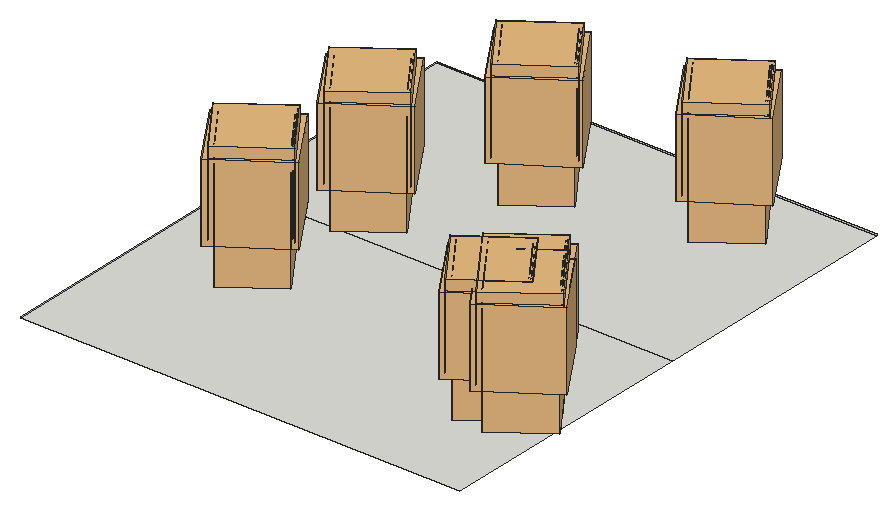
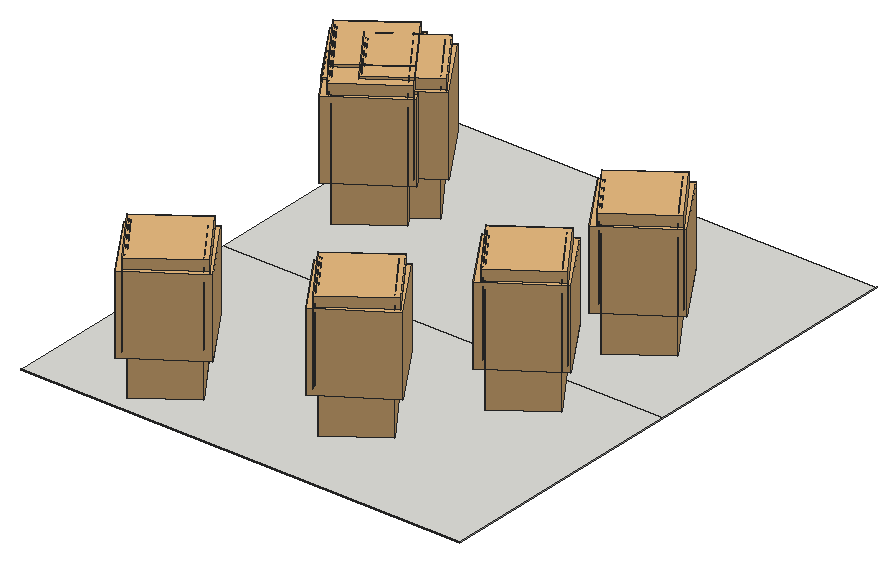
# SketchUp Ruby script. Lengths in inches.
U = 1.inch
M = Sketchup.active_model
def pt(a) = Geom::Point3d.new(a.map { |v| v * U })
def face(e, loops, mat)
  f = e.add_face(loops[0].map { |a| pt(a) })
  loops[1..].each { |l| e.add_face(l.map { |a| pt(a) }).erase! }
  f.material = f.back_material = mat if mat
  f
end
# faces: each face lists its corners as indices into pts; further lists are holes
def faces(e, pts, list, mat = nil) = list.each { |f| face(e, (f[0].is_a?(Array) ? f : [f]).map { |l| l.map { |i| pts[i] } }, mat) }
# xy, xz, yz: faces in a plane at the given z, y or x. An outline is a flat list of corners, or four numbers for a rectangle; further outlines are holes
def ring(l) = l.size == 4 ? [[l[0], l[1]], [l[2], l[1]], [l[2], l[3]], [l[0], l[3]]] : l.each_slice(2).to_a
def flat(e, list, mat, &to3) = list.each { |f| face(e, (f[0].is_a?(Array) ? f : [f]).map { |l| ring(l).map { |u, v| to3.(u, v) } }, mat) }
def xy(e, z, list, mat = nil) = flat(e, list, mat) { |x, y| [x, y, z] }
def xz(e, y, list, mat = nil) = flat(e, list, mat) { |x, z| [x, y, z] }
def yz(e, x, list, mat = nil) = flat(e, list, mat) { |y, z| [x, y, z] }
def lines(e, pts, list) = list.each { |a, b| e.add_line(pt(pts[a]), pt(pts[b])) }
# prism: a flat outline (further loops are holes) pulled along v
def prism(e, loops, v, mat = nil)
  f = face(e, loops, mat); d = Geom::Vector3d.new(v.map { |x| x * U })
  f.pushpull(f.normal.samedirection?(d) ? d.length : -d.length)
end
def box(e, o, s, mat = nil) = prism(e, [[o, [o[0] + s[0], o[1], o[2]], [o[0] + s[0], o[1] + s[1], o[2]], [o[0], o[1] + s[1], o[2]]]], [0, 0, s[2]], mat)
def at(x, y, z, deg = 0) = Geom::Transformation.translation(pt([x, y, z])) * Geom::Transformation.rotation(ORIGIN, Z_AXIS, deg.degrees)
def axes(o, x, y, z) = Geom::Transformation.new([*x, 0, *y, 0, *z, 0, *pt(o).to_a, 1])
def part(name) = M.definitions.add(name)
# library, detail: a bought-in or finely detailed component or shape, given as its bounding box
def library(name, o, s) = part(name).tap { |d| box(d.entities, o, s) }
def detail(e, o, s) = box(e.add_group.entities, o, s)
def put(e, d, t, mat = nil) = e.add_instance(d, t).tap { |i| i.material = mat if mat }
def group(e, t, mat = nil) = e.add_group.tap { |g| g.transformation = t; g.material = mat if mat }.entities
root = M.entities
M.materials.add("028_190k_fullGeometry_Material \#4").color = [120, 148, 64]
M.materials.add("Colorsadfasdfa0sd1f06w3").color = [153, 130, 61]
M.materials.add("Euphorbia asdfasd0f150160s159w").color = [180, 173, 131]
M.materials.add("Euphorbiaasdfa0sdf1a56sd016wow Leaf SU").color = [141, 134, 72]
M.materials.add("asdfasdf0165f6asdLeafVar1sfd015as60f1as6").color = [231, 235, 211]
M.materials.add("dw_stemssadfasdfa0sdf1s01d6w1").color = [90, 97, 50]
M.materials.add("viburnumblaasdfas0df1w06d").color = [98, 102, 84]
M.materials.add("viburnumbladsadfasdfad0w122").color = [125, 129, 119]
c1 = part("Component\#315")
p = [[0.25,0,0],[2.05,0.01,0.35],[1.81,4.2,1.66],[0,4.19,1.3125]]
faces(c1.entities,p,[[0,1,2,3]],"viburnumbladsadfasdfad0w122")
c2 = part("viburnumblad2")
put(c2.entities,c1,axes([-19.23,-4.49,-32.18],[83.35428,0,0],[0,79.38502,0],[0,0,83.35428]))
c3 = part("vdw_leaf\#3")
p = [[0,0,0],[-2.77,1.61,2.32],[-4.3125,6.1,4.5],[-3.97,13.49,6.09],[-2.47,18.57,6.3],[-0.2,22.73,5.75],
  [2.54,19.66,6.85],[4.3,15.93,7.09],[5.03,7.6,5.43],[3.32,1.76,2.74]]
faces(c3.entities,p,[[0,1,2,3,4,5],[0,5,6,7,8,9]],"asdfasdf0165f6asdLeafVar1sfd015as60f1as6")
c4 = part("dw_brancj_2\#2")
p = [[9.7,-0.22,29.95],[0.23,-1.96,0.34],[-0.05,1.51,0.11],[9.65,1.51,29.46],[18.64,-8.75,84.43],[18.96,-6.63,84.625],
  [1.53,6.02,63.68],[1.42,8.18,63.25],[-10.58,8.77,161.17],[-10.41,9.98,160.68],[26.34,-9.37,211.72],[26.57,-8.28,211.23]]
faces(c4.entities,p,[[0,1,2],[0,2,3],[4,0,3],[4,3,5],[6,0,3],[6,3,7],[8,6,7],[8,7,9],
  [10,4,5],[10,5,11]],"dw_stemssadfasdfa0sdf1s01d6w1")
c5 = part("vdw_branch2\#3")
put(c5.entities,c3,axes([19.53,-5.9,102.42],[1.12377,-0.50004,0],[0.46097,1.03596,0.47664],[-0.19377,-0.43548,1.13389]))
put(c5.entities,c3,axes([-5.89,6.52,109.44],[-1.07209,0.83679,0],[-0.77141,-0.98832,0.52702],[0.32427,0.41545,1.25373]))
put(c5.entities,c3,axes([-0.44,8.23,75.28],[0.88709,-0.9947,0],[0.92159,0.82189,0.33087],[-0.25219,-0.22491,1.26111]))
put(c5.entities,c3,axes([24.71,-8.97,190.81],[-0.82641,0.91101,0],[-0.83983,-0.76184,0.47664],[0.35303,0.32025,1.13389]))
put(c5.entities,c3,axes([-2.29,8.24,91.35],[1.24603,-0.47303,0],[0.43826,1.15445,0.33087],[-0.11993,-0.31592,1.26111]))
put(c5.entities,c3,axes([12.26,-3.11,37.92],[-0.64625,1.02205,0.22511],[-1.04383,-0.61044,-0.22511],[-0.07533,-0.30931,1.18809]))
put(c5.entities,c3,axes([26.17,-9.17,210.27],[-0.99452,-0.10453,0],[0.09636,-0.91681,0.38752],[-0.04051,0.38539,0.92186]))
put(c5.entities,c3,axes([-6.07,9.4,125.35],[-0.90214,-0.98107,0],[0.90896,-0.83583,0.33087],[-0.24874,0.22873,1.26111]))
put(c5.entities,c3,axes([-4.13,7.29,110.58],[0.44715,-1.078,0.64369],[1.05816,0.63649,0.33087],[-0.58725,0.40856,1.09216]))
put(c5.entities,c3,axes([23.91,-8.22,171.96],[0.62307,0.85009,-0.63406],[-0.71531,0.8798,0.47664],[0.78296,0.12729,0.94004]))
put(c5.entities,c4,at(-0.09,0.18,-0.25),"dw_stemssadfasdfa0sdf1s01d6w1")
put(c5.entities,c3,axes([23.34,-9.65,156.59],[-0.31364,-1.00782,0.58216],[1.10369,-0.17062,0.29925],[-0.17137,0.6239,0.98776]))
put(c5.entities,c3,axes([15.03,-3.37,58.83],[-1.05425,-0.00194,0.58442],[-0.14303,-1.11707,-0.26172],[0.55355,-0.3046,0.99755]))
put(c5.entities,c3,axes([-11.625,9.46,160.37],[0.36812,0.92978,0],[-0.85713,0.33936,0.38752],[0.3603,-0.14265,0.92186]))
put(c5.entities,c3,axes([21.32,-8.53,138.72],[1.21379,0.19904,0],[-0.19904,1.21379,0],[0,0,1.23]))
put(c5.entities,c3,axes([22.54,-9.2,141.43],[-1.02887,0.17955,0.60182],[-0.23387,-1.13057,-0.06253],[0.56696,-0.17376,1.02111]))
put(c5.entities,c3,axes([23.9,-8.82,173.84],[-1.14567,-0.37474,0],[0.35918,-1.0981,0.04438],[-0.01409,0.04308,1.17993]))
put(c5.entities,c3,axes([-7.84,8.92,143.59],[-1.26971,0.40522,0],[-0.37543,-1.17638,0.33087],[0.10274,0.32192,1.26111]))
put(c5.entities,c3,axes([19.77,-8.01,85.98],[-0.32405,-1.14591,0.18674],[1.10278,-0.32969,-0.10948],[0.15845,0.14442,1.16117]))
put(c5.entities,c3,axes([-0.62,5.76,76.34],[-0.08879,1.17576,-0.67771],[-1.34525,-0.16582,-0.11144],[-0.17897,0.66309,1.17383]))
put(c5.entities,c3,axes([20.49,-8.22,121.07],[0.39924,-0.78471,-0.8233],[1.08735,0.33121,0.2116],[0.09035,-0.83005,0.83495]))
put(c5.entities,c3,axes([15.15,-3.72,62.9],[1.16251,0.40128,-0.0211],[-0.39924,1.16074,0.07874],[0.0456,-0.06757,1.2273]))
put(c5.entities,c3,axes([20.72,-8.08,120.26],[-0.03693,1.2277,-0.06551],[-1.22944,-0.03698,0],[-0.00197,0.06548,1.22825]))
put(c5.entities,c3,axes([22.58,-8.36,155.57],[-0.56247,1.09386,0],[-1.00839,-0.51852,0.47664],[0.42389,0.21796,1.13389]))
put(c5.entities,c3,axes([3.97,3.13,57.96],[-1.09459,0.76041,0],[-0.72262,-1.0402,-0.1735],[-0.10109,-0.14552,1.29352]))
put(c5.entities,c3,axes([-10.8,9.06,160.75],[-0.66334,-0.72138,0],[0.66835,-0.61458,0.24329],[-0.1829,0.16818,0.92729]))
put(c5.entities,c3,axes([19.06,-9.3125,103.96],[-1.01345,0.25553,-0.60051],[-0.2265,-1.12952,-0.09839],[-0.59598,0.03076,1.01889]))
put(c5.entities,c3,axes([18.07,-6.2,81.7],[-0.56247,1.09386,0],[-1.00839,-0.51852,0.47664],[0.42389,0.21796,1.13389]))
put(c5.entities,c3,axes([12.95,-0.39,43.31],[0.13044,-1.19832,0],[1.11025,0.12085,0.29925],[-0.30382,-0.03307,1.14057]))
put(c5.entities,c3,axes([2.28,8.28,56.18],[1.32413,-0.31027,0],[0.30923,1.31968,-0.11144],[0.02542,0.1085,1.35543]))
put(c5.entities,c3,axes([-7.55,9.96,143.07],[1.34251,-0.21744,0],[0.20045,1.23761,0.52702],[-0.08426,-0.52024,1.25373]))
put(c5.entities,c3,axes([26.15,-8.25,210.66],[0.94661,-0.25364,0],[0.235,0.87703,0.24329],[-0.06431,-0.24,0.92729]))
put(c5.entities,c3,axes([-6.48,11.37,125.16],[0.64635,1.10315,0.46356],[-1.16569,0.46153,0.52702],[0.27017,-0.6478,1.16488]))
put(c5.entities,c3,axes([25.74,-8.35,191.28],[0.13044,-1.19832,0],[1.11025,0.12085,0.29925],[-0.30382,-0.03307,1.14057]))
put(c5.entities,c3,axes([-5.125,7.47,91.6],[-1.10024,0.63688,0.48318],[-0.78682,-1.00808,-0.46292],[0.14137,-0.65404,1.184]))
c6 = part("Component\#314")
p = [[0.14,0,0],[2.58,0.05,0.25],[2.44,5.11,2.64],[0,5.05,2.39]]
faces(c6.entities,p,[[0,1,2,3]],"viburnumblaasdfas0df1w06d")
c7 = part("viburnumblad1\#2")
put(c7.entities,c6,axes([-37.25,6.23,19.31],[75.98784,0,0],[0,65.50676,0],[0,0,75.98784]))
c8 = part("vdw_leaf\#2")
p = [[0,0,0],[-2.77,1.61,2.32],[-4.3125,6.1,4.5],[-3.97,13.49,6.09],[-2.47,18.57,6.3],[-0.2,22.73,5.75],
  [2.54,19.66,6.85],[4.3,15.93,7.09],[5.03,7.6,5.43],[3.32,1.76,2.74]]
faces(c8.entities,p,[[0,1,2,3,4,5],[0,5,6,7,8,9]],"asdfasdf0165f6asdLeafVar1sfd015as60f1as6")
c9 = part("dg_branch_1\#2")
p = [[46.12,1.57,35.62],[46,5.42,35.41],[0.14,1.79,0.05],[0.26,-2.0625,0.27],[74.05,2.99,75.8],[74.11,5.28,75.58],
  [103.46,0.47,94.74],[104.03,2.92,94.84],[81.14,16.92,120.46],[81.2,18.78,120.24],[130.47,-5.6875,130.27],[130.58,-3.66,129.85],
  [80.82,34.4375,191.22],[80.64,35.93,190.9],[148.49,-14.56,203.24],[148.9,-12.8125,203.11],[81.08,37.95,226.93],[81.4,39.1,227.03],
  [157.45,-18.19,250.77],[157.7,-17.01,250.41]]
faces(c9.entities,p,[[0,1,2,3],[4,0,1],[4,1,5],[6,4,5],[6,5,7],[8,4,5],[8,5,9],[10,6,7],
  [10,7,11],[12,8,9],[12,9,13],[14,10,11],[14,11,15],[16,12,13],[16,13,17],[18,14,15],
  [18,15,19]],"dw_stemssadfasdfa0sdf1s01d6w1")
c10 = part("vdw_branch1\#3")
put(c10.entities,c8,axes([120.69,-2.42,117.31],[1.12221,-0.24063,-0.65809],[0.19207,1.24776,-0.12871],[0.65778,0.01392,1.11658]))
put(c10.entities,c8,axes([81,38.9,226.05],[0.7888,-0.58155,0],[0.48308,0.65523,0.47],[-0.28484,-0.38635,0.83138]))
put(c10.entities,c8,axes([78.08,12.69,106.05],[-1.43826,-0.02353,-0.03177],[0.0088,-1.31777,0.57755],[-0.03854,0.57714,1.31741]))
put(c10.entities,c8,axes([130.18,-4.73,130.41],[-0.38031,-1.29044,-0.11242],[1.20662,-0.31032,-0.51987],[0.47109,-0.24694,1.24081]))
put(c10.entities,c8,axes([157.08,-17.89,249.93],[-0.91355,0.40674,0],[-0.37496,-0.84216,0.38752],[0.15762,0.35401,0.92186]))
put(c10.entities,c8,axes([90.64,3.03,86.49],[0.32514,-0.85045,-0.99675],[0.69523,0.98247,-0.61148],[1.11061,-0.36604,0.67459]))
put(c10.entities,c8,axes([80.15,28.42,160.95],[-0.16039,0.95636,-1.06292],[-1.41646,0.03966,0.24943],[0.19509,1.07422,0.93709]))
put(c10.entities,c8,axes([126.74,-5.45,129.22],[-0.59819,0.96152,-0.6841],[-0.85772,0.12575,0.92675],[0.75427,0.88089,0.57856]))
put(c10.entities,c8,axes([133.22,-6.12,150.66],[-0.93823,0.76985,0.59124],[-0.47726,-1.08188,0.65135],[0.84525,0.24366,1.02405]))
put(c10.entities,c8,axes([80.43,22.89,141.32],[-1.42571,-0.19312,0.01373],[0.18338,-1.31425,0.5561],[-0.0621,0.5528,1.32692]))
put(c10.entities,c8,axes([33.14,0.88,26.42],[-0.13338,1.31536,0.04876],[-1.04528,-0.13221,0.7073],[0.72315,0.03348,1.07497]))
put(c10.entities,c8,axes([152.63,-15.08,221.76],[-1.28188,0.41945,0.0579],[-0.3638,-1.18547,0.53367],[0.21665,0.49113,1.23869]))
put(c10.entities,c8,axes([80.05,28.28,160.33],[-0.46732,-1.26661,0.40679],[1.27397,-0.40257,0.21004],[-0.07408,0.44645,1.30501]))
put(c10.entities,c8,axes([153.95,-14.8,235.875],[0.39005,1.07743,0.20605],[-0.96443,0.25296,0.50293],[0.42961,-0.3464,0.99807]))
put(c10.entities,c8,axes([80.2,24.22,141.74],[1.33062,-0.46576,0.02628],[0.44746,1.2746,-0.06608],[-0.00197,0.0722,1.37936]))
put(c10.entities,c8,axes([145.48,-12.5,188.92],[-1.32952,0.16983,0.16138],[-0.09299,-1.2361,0.53471],[0.21503,0.51548,1.22904]))
put(c10.entities,c8,axes([139.64,-9.18,171.24],[0.05682,1.30088,0.23414],[-1.13176,-0.05343,0.57151],[0.58357,-0.22963,1.13417]))
put(c10.entities,c8,axes([70.95,4.35,71.98],[-1.1081,-0.41873,0.64752],[0.33675,-1.28259,-0.25313],[0.6937,-0.04625,1.15721]))
put(c10.entities,c8,axes([59.85,4.55,56.17],[-0.26797,1.24526,0.35754],[-0.9369,-0.41634,0.74783],[0.83377,-0.10389,0.98674]))
put(c10.entities,c8,axes([33.11,3.36,25.66],[-0.57817,-1.07968,-0.5679],[1.11554,-0.21356,-0.7297],[0.49375,-0.78178,0.98363]))
put(c10.entities,c9,at(-0.21,0.34,-0.17),"dw_stemssadfasdfa0sdf1s01d6w1")
put(c10.entities,c8,axes([80.91,19.01,122.53],[-0.84258,1.13222,-0.27981],[-1.15093,-0.75138,0.42537],[0.18861,0.47293,1.3457]))
put(c10.entities,c8,axes([119.8,-1.22,114.1],[-1.3235,-0.25012,0.09101],[0.25933,-1.31572,0.15537],[0.05991,0.1698,1.33794]))
put(c10.entities,c8,axes([46.29,5.1,38.04],[0.98937,0.73827,-0.47585],[-0.72359,1.03721,0.10473],[0.44068,0.18581,1.20453]))
put(c10.entities,c8,axes([81.1875,33.03,184.45],[1.33883,0.26986,0.35053],[-0.09581,1.22087,-0.57399],[-0.42216,0.53228,1.20262]))
put(c10.entities,c8,axes([80.16,36.28,206.98],[-0.83993,0.85737,-0.6234],[-1.05964,-0.65701,0.5241],[0.02941,0.81391,1.07976]))
put(c10.entities,c8,axes([154.86,-16.15,234.87],[0.02509,-1.15302,-0.28506],[1.1487,-0.04894,0.29908],[-0.30202,-0.28195,1.11384]))
put(c10.entities,c8,axes([108.77,-0.33,101.14],[-0.47691,-1.03266,-0.72709],[1.25395,-0.29455,-0.40416],[0.15052,-0.81814,1.06325]))
put(c10.entities,c8,axes([89.79,3.01,85.87],[-0.61344,0.75518,0.8965],[-0.17758,-1.01824,0.73622],[1.13385,0.22574,0.58569]))
put(c10.entities,c8,axes([81.56,20.31,123.29],[0.37259,-1.3435,0.21057],[1.29385,0.32364,-0.22445],[0.16906,0.25791,1.34638]))
put(c10.entities,c8,axes([46.45,1.82,36.74],[-0.77883,0.29892,1.0614],[0.19124,-1.24314,0.49044],[1.08598,0.43329,0.67484]))
put(c10.entities,c8,axes([71.37,4.02,72.32],[0.72905,0.81546,-0.74421],[-0.66805,0.98958,0.42988],[0.8391,0.14186,0.97745]))
put(c10.entities,c8,axes([136.59,-5.88,150.53],[0.85845,-0.99897,-0.12437],[0.96526,0.81273,0.13453],[-0.02572,-0.18182,1.28292]))
put(c10.entities,c8,axes([80.375,38.8,225.86],[-0.25178,0.96778,0],[-0.89216,-0.23211,0.38752],[0.37503,0.09757,0.92186]))
put(c10.entities,c8,axes([74.43,7.99,85.38],[-1.05703,0.91669,-0.33543],[-0.95806,-0.87958,0.61531],[0.18697,0.6754,1.25659]))
put(c10.entities,c8,axes([76.57,9.74,89.32],[0.63146,-1.21538,0.33508],[1.18148,0.49387,-0.43517],[0.26321,0.48577,1.26593]))
put(c10.entities,c8,axes([81.6875,36.97,207.4],[0.09422,-1.04424,0.38486],[1.01646,0.1939,0.27727],[-0.33299,0.33382,0.98727]))
put(c10.entities,c8,axes([157.29,-17.17,249.98],[0.50586,-0.50586,0],[0.38853,0.38853,0.41105],[-0.29684,-0.29684,0.56115]))
put(c10.entities,c8,axes([79.92,15.8,106.09],[1.03917,-0.29343,-0.90675],[-0.14587,1.22131,-0.5624],[0.92163,0.5191,0.88824]))
put(c10.entities,c8,axes([61.95,3.88,56.26],[0.41243,-1.28546,0],[1.17466,0.37688,-0.54831],[0.5221,0.16751,1.23363]))
put(c10.entities,c8,axes([151.99,-14.79,208.15],[-0.48571,-1.21723,-0.32393],[1.25386,-0.50033,0],[-0.12005,-0.30087,1.31056]))
put(c10.entities,c8,axes([108.44,0.62,102.22],[0.82183,0.96078,0.38967],[-0.62327,0.08618,1.10203],[0.79141,-0.88661,0.51693]))
put(c10.entities,c8,axes([145.6,-10.56,188.62],[1.03241,-0.02554,-0.82693],[0.3944,1.11584,0.45794],[0.70325,-0.61672,0.89706]))
put(c10.entities,c8,axes([78.59,32.3,183.89],[-1.12675,-0.42036,0.43987],[0.5899,-0.98149,0.57312],[0.14901,0.70693,1.05726]))
put(c10.entities,c8,axes([152.08,-13.42,223.37],[0.79993,-0.44251,-0.69938],[0.68456,0.82615,0.26026],[0.41048,-0.60953,0.85515]))
put(c10.entities,c8,axes([140.71,-8.74,170.55],[0.41903,-1.24177,-0.32393],[1.26224,0.33728,0.33986],[-0.23168,-0.40836,1.26573]))
put(c10.entities,c8,axes([149.25,-12.53,205.78],[1.24456,0.38285,0.23414],[-0.42999,1.04826,0.57151],[-0.02056,-0.62679,1.13417]))
c11 = part("Component\#306")
p = [[4.55,0.11,0],[4.55,0,0],[2.84,0,3.13],[2.84,0.11,3.13],[4.625,0.05,0.04],[2.92,0.05,3.15],
  [2.08,0,8.07],[2.08,0.11,8.07],[2.16,0.05,8.1],[0,0,12.54],[0,0.11,12.54],[0.07,0.05,12.58]]
faces(c11.entities,p,[[0,1,2,3],[1,4,5,2],[1,0,4],[4,0,3,5],[3,2,6,7],[2,5,8,6],[5,3,7,8],[7,6,9,10],
  [6,8,11,9],[8,7,10,11],[10,9,11]],"Colorsadfasdfa0sd1f06w3")
c12 = part("Component\#301")
xy(c12.entities,0,[[0,0,0.7,3.1]],"Euphorbiaasdfa0sdf1a56sd016wow Leaf SU")
c13 = part("Leaf rosette")
put(c13.entities,c12,axes([2.21,1.74,0.13],[-0.4441,0.47879,-0.0956],[-0.4878,-0.4406,0.05935],[-0.03146,0.16757,0.98536]))
put(c13.entities,c12,axes([2.29,1.9,0.17],[-0.62678,-0.10063,-0.18061],[0.01105,-0.59203,0.2915],[-0.31282,0.41486,0.85442]))
put(c13.entities,c12,axes([2.09,1.69,0.1],[-0.10438,0.65169,0],[-0.65169,-0.10438,0],[0,0,1]))
put(c13.entities,c12,axes([1.97,1.77,0.02],[0.31114,0.5228,0.25587],[-0.57125,0.32993,0.02052],[-0.16918,-0.3502,0.92127]))
put(c13.entities,c12,axes([1.93,1.95,0],[0.54816,-0.03215,0.36617],[-0.11878,0.60671,0.23108],[-0.52706,-0.39065,0.75472]))
put(c13.entities,c12,axes([2.04,2.1,0.05],[0.26275,-0.55867,0.23335],[0.34186,0.34684,0.44545],[-0.75711,-0.08556,0.64766]))
put(c13.entities,c12,axes([2.22,2.08,0.13],[-0.29265,-0.59104,-0.02512],[0.40323,-0.2198,0.47401],[-0.65583,0.2952,0.69479]))
c14 = part("Component\#308")
xy(c14.entities,0,[[0,0,5.01,4.64]],"Euphorbia asdfasd0f150160s159w")
c15 = part("Component\#316")
put(c15.entities,c11,at(2.35,3.5,0))
put(c15.entities,c13,at(0.25,1.59,12.45))
put(c15.entities,c14,axes([7.46,0.77,3.64],[0.10848,0.99337,0.03799],[-0.82378,0.11122,-0.55589],[-0.55643,0.02901,0.83038]))
put(c15.entities,c14,axes([1.97,2.58,1.93],[0.80762,-0.50565,0.30344],[0.47433,0.86274,0.17519],[-0.35038,0.00244,0.93661]))
put(c15.entities,c14,axes([5.79,0.14,3.9],[0.5013,0.78918,0.35482],[-0.74775,0.60146,-0.2813],[-0.4354,-0.1243,0.89162]))
put(c15.entities,c14,axes([1.87,2.6,3.75],[0.73154,-0.49698,0.46676],[0.47433,0.86274,0.17519],[-0.48976,0.09324,0.86686]))
put(c15.entities,c14,axes([3.91,7.06,6.66],[-0.50827,-0.83837,-0.19699],[0.8278,-0.53869,0.15675],[-0.23753,-0.08339,0.96779]))
put(c15.entities,c14,axes([1.2,3.99,6.83],[0.56066,-0.79708,0.22433],[0.74237,0.60386,0.29025],[-0.36682,0.0038,0.93028]))
put(c15.entities,c12,axes([2.42,3.73,12.57],[-0.1322,-0.64472,0.04955],[0.10064,0.02944,0.65162],[-0.9678,0.2092,0.14002]))
put(c15.entities,c12,axes([2.57,3.43,12.63],[-0.62833,0.089,-0.18134],[-0.19954,-0.36568,0.51192],[-0.04764,0.82148,0.56824]))
put(c15.entities,c14,axes([4.04,6.92,11.09],[-0.67411,-0.5063,-0.5378],[0.44628,-0.85937,0.24964],[-0.58857,-0.07172,0.80526]))
put(c15.entities,c12,axes([2.5,3.49,12.74],[-0.62833,0.089,-0.18134],[-0.18746,-0.03618,0.63178],[0.11402,0.98935,0.09049]))
put(c15.entities,c12,axes([2.3,3.27,12.51],[0.02916,0.64747,0.12464],[-0.56235,-0.04072,0.34308],[0.5216,-0.18387,0.83314]))
put(c15.entities,c14,axes([0.26,4.96,9.69],[0.33661,-0.92735,0.16343],[0.73504,0.36725,0.56995],[-0.58857,-0.07172,0.80526]))
put(c15.entities,c14,axes([4.76,6.31,12.62],[-0.95056,-0.1129,-0.28929],[0.09021,-0.99179,0.09066],[-0.29715,0.06008,0.95294]))
put(c15.entities,c14,axes([5.2,6.55,10.37],[-0.76372,-0.27738,-0.58291],[0.26517,-0.95808,0.10848],[-0.58857,-0.07172,0.80526]))
c16 = part("Plant stem")
p = [[2.84,0.11,3.13],[2.84,0,3.13],[2.08,0,8.07],[2.08,0.11,8.07],[2.92,0.05,3.15],[2.16,0.05,8.1],
  [0,0,12.54],[0,0.11,12.54],[0.07,0.05,12.58]]
faces(c16.entities,p,[[0,1,2,3],[1,4,5,2],[4,0,3,5],[3,2,6,7],[2,5,8,6],[5,3,7,8],[7,6,8]],"Colorsadfasdfa0sd1f06w3")
c17 = part("Leafy shoot")
put(c17.entities,c16,at(2.35,3.5,0))
put(c17.entities,c13,at(0.25,1.59,12.45))
put(c17.entities,c14,axes([1.87,2.6,3.75],[0.73154,-0.49698,0.46676],[0.47433,0.86274,0.17519],[-0.48976,0.09324,0.86686]))
put(c17.entities,c14,axes([3.91,7.06,6.66],[-0.50827,-0.83837,-0.19699],[0.8278,-0.53869,0.15675],[-0.23753,-0.08339,0.96779]))
put(c17.entities,c14,axes([1.2,3.99,6.83],[0.56066,-0.79708,0.22433],[0.74237,0.60386,0.29025],[-0.36682,0.0038,0.93028]))
put(c17.entities,c12,axes([2.42,3.73,12.57],[-0.1322,-0.64472,0.04955],[0.10064,0.02944,0.65162],[-0.9678,0.2092,0.14002]))
put(c17.entities,c12,axes([2.57,3.43,12.63],[-0.62833,0.089,-0.18134],[-0.19954,-0.36568,0.51192],[-0.04764,0.82148,0.56824]))
put(c17.entities,c14,axes([4.04,6.92,11.09],[-0.67411,-0.5063,-0.5378],[0.44628,-0.85937,0.24964],[-0.58857,-0.07172,0.80526]))
put(c17.entities,c12,axes([2.5,3.49,12.74],[-0.62833,0.089,-0.18134],[-0.18746,-0.03618,0.63178],[0.11402,0.98935,0.09049]))
put(c17.entities,c12,axes([2.3,3.27,12.51],[0.02916,0.64747,0.12464],[-0.56235,-0.04072,0.34308],[0.5216,-0.18387,0.83314]))
put(c17.entities,c14,axes([0.26,4.96,9.69],[0.33661,-0.92735,0.16343],[0.73504,0.36725,0.56995],[-0.58857,-0.07172,0.80526]))
put(c17.entities,c14,axes([4.76,6.31,12.62],[-0.95056,-0.1129,-0.28929],[0.09021,-0.99179,0.09066],[-0.29715,0.06008,0.95294]))
put(c17.entities,c14,axes([5.2,6.55,10.37],[-0.76372,-0.27738,-0.58291],[0.26517,-0.95808,0.10848],[-0.58857,-0.07172,0.80526]))
put(c17.entities,c14,axes([7.03,0.77,3.77],[0.19714,0.84663,0.32426],[-0.94994,0.28899,-0.30484],[-0.2731,-0.45173,0.91532]))
c18 = part("Groundcover plant")
put(c18.entities,c15,axes([0.82,1.83,0.8125],[0.98541,0,-0.17021],[0,1,0],[0.17021,0,0.98541]))
put(c18.entities,c17,axes([4.45,-0.84,-2.24],[0.69527,0.50616,0],[-0.50264,0.69042,-0.10135],[-0.05965,0.08194,0.85401]))
put(c18.entities,c17,axes([1.85,7.37,-3.38],[0.7038,-0.47341,0.14191],[0.46407,0.71797,0.09357],[-0.16999,0,0.84303]))
put(c18.entities,c17,axes([6.9,-3.65,-2.52],[0.79351,0.57769,0],[-0.57366,0.78798,-0.11567],[-0.06808,0.09351,0.97468]))
put(c18.entities,c17,axes([1.36,5.18,-2.66],[0.50674,-0.34086,0.10218],[0.33413,0.51694,0.06737],[-0.12239,0,0.60698]))
put(c18.entities,c17,axes([5.76,-1.49,-2.17],[0.43479,0.43181,0.07251],[-0.43488,0.43544,-0.06951],[-0.06212,-0.06169,0.61918]))
c19 = part("Groundcover clump")
put(c19.entities,c18,axes([25.06,6.72,0.82],[-0.74291,1.22188,0],[-1.22188,-0.74291,0],[0,0,1]))
put(c19.entities,c18,axes([-0.76,2.1875,0.82],[1.43,0,0],[0,1.43,0],[0,0,1]))
put(c19.entities,c18,axes([8.21,24.79,0.82],[-0.6403,-1.27864,0],[1.27864,-0.6403,0],[0,0,1]))
c20 = library("028_190k_fullGeometry_0",[-319.99,-281.1,-2.15],[577.33,562.38,1159.36])
c21 = library("028_190k_fullGeometry_1",[-333.4,-281.7,421.48],[600.33,578.53,738.83])
c22 = library("028_190k_fullGeometry_2",[-3584003,-3264710,4041818.25],[6566285.5,6460741.75,7903602.75])
c23 = library("028_190k_fullGeometry_3",[-353.86,-324.57,405.22],[652.24,636.69,781.83])
c24 = part("028_190k_fullGeometry_4")
p = [[125.51,152.8,882.93],[125.36,152.82,883.01],[124.8,155.5625,881.05]]
faces(c24.entities,p,[[0,1,2]],"028_190k_fullGeometry_Material \#4")
c25 = part("028_190k_fullGeometry")
g1 = group(c25.entities,at(0,0,0))
put(g1,c20,axes([0,0,0],[0.18998,-0.26642,0],[0.26642,0.18998,0],[0,0,0.32722]))
put(g1,c21,axes([0,0,0],[0.18998,-0.26642,0],[0.26642,0.18998,0],[0,0,0.32722]))
put(g1,c22,axes([0,0,0],[0.00002,-0.00003,0],[0.00003,0.00002,0],[0,0,0.00003]))
put(g1,c23,axes([0,0,0],[0.18998,-0.26642,0],[0.26642,0.18998,0],[0,0,0.32722]))
put(g1,c24,axes([0,0,0],[0.18998,-0.26642,0],[0.26642,0.18998,0],[0,0,0.32722]))
xy(root,-9,[[0,0,1338.625,807.5],[0,807.5,1338.625,1583.3125]])
xz(root,1583.3125,[[0,-9,1338.625,-6]])
yz(root,0,[[0,-9,1583.3125,-6]])
put(root,c2,axes([1228.01,298.625,25.32],[0.00025,0.00856,-0.00655],[-0.01174,-0.00053,-0.00107],[-0.00121,0.00703,0.00818]))
put(root,c2,axes([1225.36,297.64,11.8125],[0.01065,0.00175,0.00643],[0.00257,0.00902,-0.00671],[-0.00605,0.00763,0.00794]))
put(root,c2,axes([1230.07,299.18,28.21],[0.00655,-0.0105,0.00435],[0.00979,0.0053,-0.00197],[-0.0002,0.0047,0.01165]))
put(root,c2,axes([1228.48,300.84,25.5],[-0.00824,-0.00797,0.00286],[0.00803,-0.0057,0.00726],[-0.00361,0.00659,0.00792]))
put(root,c2,axes([1228.51,300.97,27.11],[-0.01151,-0.00126,-0.00215],[-0.00046,-0.00922,0.00721],[-0.00262,0.00705,0.00788]))
put(root,c5,axes([1200.82,295.23,1.63],[0.02088,0.1592,-0.03733],[-0.16201,0.02125,0],[0.00395,0.03008,0.19757]))
put(root,c7,axes([1230.96,299.42,20.27],[-0.01249,0.00074,0.00321],[0.00342,-0.00484,0.01344],[0.00175,0.01171,0.00271]))
put(root,c2,axes([1238.65,300.51,22.34],[-0.01262,0.00712,0.00249],[-0.00199,-0.00788,0.01243],[0.00728,0.01023,0.00765]))
put(root,c2,axes([1228.09,300.2,24.22],[-0.00014,-0.00961,0.00594],[0.01198,0.00212,0.00345],[-0.00404,0.00568,0.00838]))
put(root,c2,axes([1224.63,298.35,13.27],[0.01002,0.00748,-0.00127],[-0.0057,0.00603,-0.00944],[-0.00501,0.0081,0.0082]))
put(root,c2,axes([1229.53,297.83,28.86],[0.01039,0.00506,-0.00344],[-0.00658,0.01149,-0.00298],[0.00188,0.00411,0.01172]))
put(root,c7,axes([1229.23,297.58,25.53],[0.0119,-0.00534,0.00444],[0.00766,0.01326,-0.00459],[-0.00215,0.00555,0.01243]))
put(root,c2,axes([1225.3,299.48,12.39],[0.00504,-0.005,0.01036],[0.00925,0.00849,-0.00041],[-0.00684,0.0078,0.00709]))
put(root,c2,axes([1227.32,300.11,27.34],[0.00014,0.01001,-0.00619],[-0.01174,-0.00053,-0.00107],[-0.00123,0.00599,0.0089]))
put(root,c2,axes([1237.66,302.09,21.4375],[-0.00284,-0.00899,0.01128],[0.01228,-0.00546,-0.00125],[0.00539,0.01,0.00933]))
put(root,c2,axes([1236.38,301.09,20.65],[0.00722,-0.01189,0.00649],[0.01053,0.00219,-0.0077],[0.0056,0.00897,0.01021]))
put(root,c2,axes([1239.36,302.42,22.89],[-0.01093,-0.00132,0.00974],[0.00771,-0.01018,0.00728],[0.00609,0.01052,0.00826]))
put(root,c2,axes([1226.94,299.51,25.96],[0.00824,0.00797,-0.00286],[-0.00838,0.00693,-0.00484],[-0.00165,0.00508,0.00936]))
put(root,c7,axes([1234.05,298.73,18.83],[0.01385,-0.00786,0.00256],[0.00839,0.01058,-0.01294],[0.00399,0.01072,0.01136]))
put(root,c2,axes([1230.66,301.67,21.88],[-0.01171,0.00153,-0.0034],[-0.00332,-0.0036,0.00923],[0.00008,0.01052,0.00323]))
put(root,c2,axes([1227.69,301.91,26.32],[-0.00014,-0.01001,0.00619],[0.0111,0.00196,0.00319],[-0.00404,0.00568,0.00838]))
put(root,c2,axes([1227.18,300.81,25.22],[0.00804,-0.00619,0.0059],[0.00785,0.00862,-0.00178],[-0.00364,0.00486,0.00899]))
put(root,c2,axes([1230.09,302.27,20.65],[-0.00352,-0.00505,0.00939],[0.01197,-0.00026,0.00408],[-0.00173,0.01006,0.00403]))
put(root,c7,axes([1227.07,301.01,28.62],[-0.00083,0.01216,-0.00686],[-0.01618,-0.00142,-0.00053],[-0.00101,0.00652,0.01095]))
put(root,c2,axes([1238.73,301.45,24.35],[-0.00691,0.01139,-0.00621],[-0.01,-0.00019,0.01077],[0.00826,0.00929,0.00783]))
put(root,c2,axes([1235.86,300,22.07],[0.01049,0.00127,-0.00935],[-0.00649,0.01342,-0.00547],[0.00778,0.00774,0.00978]))
put(root,c2,axes([1229.46,301.52,22.29],[0.00325,0.00384,-0.00943],[-0.01118,0.00267,-0.00269],[0.00139,0.01021,0.00373]))
put(root,c2,axes([1237.14,300.57,23.46],[0.00284,0.00899,-0.01128],[-0.01167,0.00819,0.00358],[0.00847,0.00827,0.00872]))
put(root,c2,axes([1230.6875,303.31,21.54],[-0.01052,-0.00268,0.00462],[0.00552,-0.00368,0.01018],[-0.00102,0.01046,0.0033]))
put(root,c2,axes([1226.49,301.05,26.55],[0.01151,0.00126,0.00215],[-0.00018,0.01065,-0.00509],[-0.00265,0.00461,0.00939]))
put(root,c2,axes([1230.36,302.66,22.71],[-0.00534,0.00476,-0.00922],[-0.00963,-0.00133,0.0047],[0.00092,0.0102,0.00386]))
put(root,c2,axes([1236.45,301.84,22.65],[0.01262,-0.00712,-0.00249],[0.00385,0.01054,-0.01059],[0.00659,0.00804,0.0104]))
put(root,c2,axes([1237.85,303.5,22.96],[0.00691,-0.01139,0.00621],[0.0117,0.00243,-0.00856],[0.0056,0.00897,0.01021]))
put(root,c2,axes([1230.77,304.1875,22.88],[-0.01122,0.00147,-0.00326],[-0.00368,-0.004,0.01025],[0.00008,0.01052,0.00323]))
put(root,c2,axes([1229.46,303.54,21.09],[0.00534,-0.00476,0.00922],[0.0104,0.00387,-0.00404],[-0.00165,0.00955,0.00498]))
put(root,c2,axes([1228.78,302.9,22.26],[0.01052,0.00268,-0.00462],[-0.0054,0.00599,-0.0087],[0.00028,0.0093,0.00555]))
put(root,c2,axes([1230.33,304.84,21.63],[-0.00367,-0.00526,0.00978],[0.01109,-0.00025,0.00378],[-0.00173,0.01006,0.00403]))
put(root,c2,axes([1237.23,302.53,24.42],[0.01093,0.00132,-0.00974],[-0.00601,0.01242,-0.00506],[0.00778,0.00774,0.00978]))
put(root,c10,axes([1198.8,293.53,0.51],[-0.01089,0.12699,0],[-0.12699,-0.01089,0],[0,0,0.15683]))
put(root,c2,axes([1229.34,303.96,23.25],[0.00367,0.00526,-0.00978],[-0.01118,0.00267,-0.00269],[0.001,0.0097,0.00482]))
put(root,c19,axes([1190.15,287.37,1.17],[1.49047,0,0],[0,1.49047,0],[0,0,1.49047]))
put(root,c2,axes([1228.91,304.61,22.01],[0.01122,-0.00147,0.00326],[0.00359,0.00643,-0.00917],[-0.00081,0.00924,0.00561]))
put(root,c25,at(1143.51,365.45,0.7))
put(root,c25,at(1237.28,365.45,0.7))
put(root,c25,at(1188.83,432.88,-5.3))
put(root,c25,at(293.26,524.51,-5.3))
put(root,c25,at(339.28,908.33,-5.3))
put(root,c25,at(570.89,1256.29,-5.3))
put(root,c25,at(1039.625,1396.26,-5.3))
